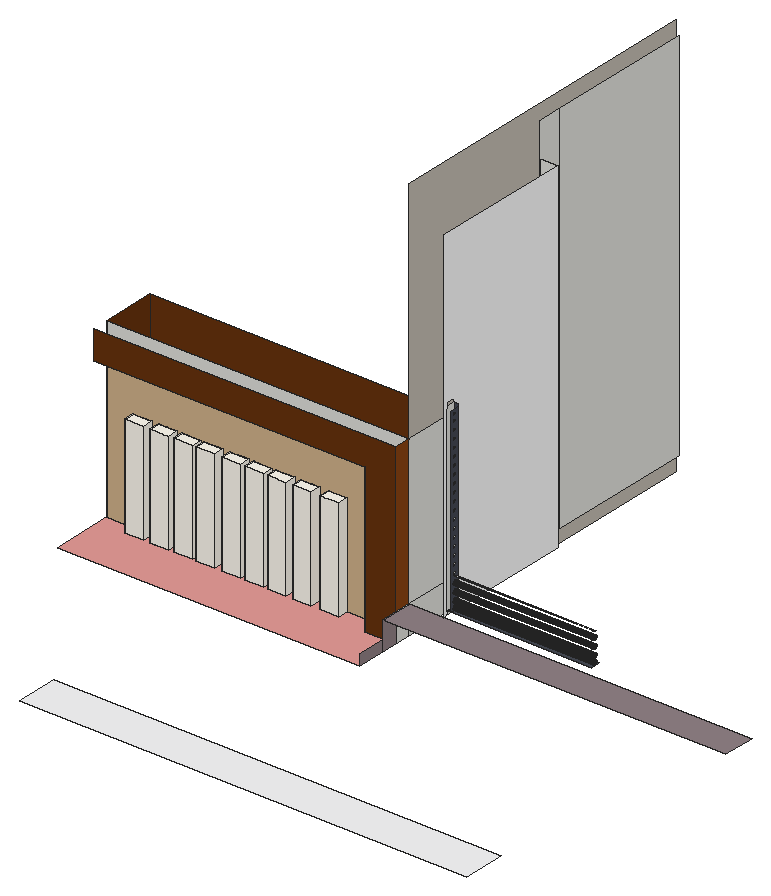
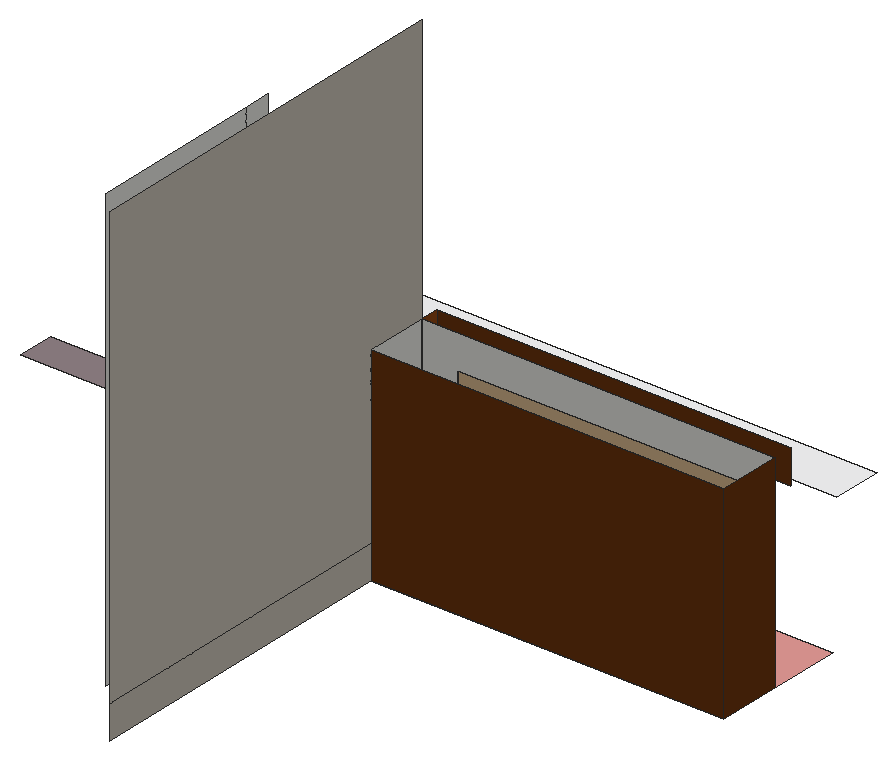
# SketchUp Ruby script. Lengths in inches.
U = 1.inch
M = Sketchup.active_model
def pt(a) = Geom::Point3d.new(a.map { |v| v * U })
def face(e, loops, mat)
  f = e.add_face(loops[0].map { |a| pt(a) })
  loops[1..].each { |l| e.add_face(l.map { |a| pt(a) }).erase! }
  f.material = f.back_material = mat if mat
  f
end
# faces: each face lists its corners as indices into pts; further lists are holes
def faces(e, pts, list, mat = nil) = list.each { |f| face(e, (f[0].is_a?(Array) ? f : [f]).map { |l| l.map { |i| pts[i] } }, mat) }
# xy, xz, yz: faces in a plane at the given z, y or x. An outline is a flat list of corners, or four numbers for a rectangle; further outlines are holes
def ring(l) = l.size == 4 ? [[l[0], l[1]], [l[2], l[1]], [l[2], l[3]], [l[0], l[3]]] : l.each_slice(2).to_a
def flat(e, list, mat, &to3) = list.each { |f| face(e, (f[0].is_a?(Array) ? f : [f]).map { |l| ring(l).map { |u, v| to3.(u, v) } }, mat) }
def xy(e, z, list, mat = nil) = flat(e, list, mat) { |x, y| [x, y, z] }
def xz(e, y, list, mat = nil) = flat(e, list, mat) { |x, z| [x, y, z] }
def yz(e, x, list, mat = nil) = flat(e, list, mat) { |y, z| [x, y, z] }
def lines(e, pts, list) = list.each { |a, b| e.add_line(pt(pts[a]), pt(pts[b])) }
# prism: a flat outline (further loops are holes) pulled along v
def prism(e, loops, v, mat = nil)
  f = face(e, loops, mat); d = Geom::Vector3d.new(v.map { |x| x * U })
  f.pushpull(f.normal.samedirection?(d) ? d.length : -d.length)
end
def box(e, o, s, mat = nil) = prism(e, [[o, [o[0] + s[0], o[1], o[2]], [o[0] + s[0], o[1] + s[1], o[2]], [o[0], o[1] + s[1], o[2]]]], [0, 0, s[2]], mat)
def at(x, y, z, deg = 0) = Geom::Transformation.translation(pt([x, y, z])) * Geom::Transformation.rotation(ORIGIN, Z_AXIS, deg.degrees)
def axes(o, x, y, z) = Geom::Transformation.new([*x, 0, *y, 0, *z, 0, *pt(o).to_a, 1])
def part(name) = M.definitions.add(name)
# library, detail: a bought-in or finely detailed component or shape, given as its bounding box
def library(name, o, s) = part(name).tap { |d| box(d.entities, o, s) }
def detail(e, o, s) = box(e.add_group.entities, o, s)
def put(e, d, t, mat = nil) = e.add_instance(d, t).tap { |i| i.material = mat if mat }
def group(e, t, mat = nil) = e.add_group.tap { |g| g.transformation = t; g.material = mat if mat }.entities
root = M.entities
M.materials.add("[0027_PeachPuff]").color = [255, 218, 185]
M.materials.add("[0035_Tan]").color = [210, 180, 140]
M.materials.add("[0043_SaddleBrown]").color = [104, 51, 14]
M.materials.add("[0043_SaddleBrown]1").color = [139, 69, 19]
M.materials.add("[0052_FloralWhite]").color = [255, 250, 240]
M.materials.add("[Asphalt New]").color = [145, 130, 134]
M.materials.add("[Brick Basket]").color = [230, 156, 152]
M.materials.add("[Field Rectangle Tile]").color = [196, 189, 179]
M.materials.add("[Formica Laminate Dark]").color = [70, 74, 84]
M.materials.add("[Polished Concrete New]").color = [200, 200, 203]
M.materials.add("[Quartz Light Grey]").color = [251, 251, 252]
xy(root,0,[[86.375,112.04,96.16,117.35],[8.39,113.98,14.33,117.35],[16.46,113.98,22.4,117.35],[23.96,113.98,29.9,117.35],[30.96,113.98,36.9,117.35],
  [39.27,113.98,45.21,117.35],[46.71,113.98,52.65,117.35],[53.83,113.98,59.77,117.35],[61.83,113.98,67.77,117.35],[70.58,113.98,76.52,117.35],
  [0,117.35,96.16,134.6]])
xy(root,0,[[0,97.66,0,117.35,8.39,117.35,8.39,113.98,14.33,113.98,14.33,117.35,16.46,117.35,16.46,113.98,22.4,113.98,22.4,117.35,23.96,117.35,23.96,113.98,29.9,113.98,29.9,117.35,30.96,117.35,30.96,113.98,36.9,113.98,36.9,117.35,39.27,117.35,39.27,113.98,45.21,113.98,45.21,117.35,46.71,117.35,46.71,113.98,52.65,113.98,52.65,117.35,53.83,117.35,53.83,113.98,59.77,113.98,59.77,117.35,61.83,117.35,61.83,113.98,67.77,113.98,67.77,117.35,70.58,117.35,70.58,113.98,76.52,113.98,76.52,117.35,86.375,117.35,86.375,112.04,96.16,112.04,96.16,97.66]],"[Brick Basket]")
xy(root,0,[[41.43,31,183.87,44.5]],"[Quartz Light Grey]")
xy(root,9,[[96.16,107.04,205.34,117.35]],"[Asphalt New]")
xy(root,10.25,[[107.21,118.87,108.27,121.64]])
xy(root,10.25,[[108.27,118.87,153.22,121.64]],"[Formica Laminate Dark]")
xy(root,32.4375,[[8.39,113.98,14.33,117.35],[16.46,113.98,22.4,117.35],[23.96,113.98,29.9,117.35],[30.96,113.98,36.9,117.35],[39.27,113.98,45.21,117.35],
  [46.71,113.98,52.65,117.35],[53.83,113.98,59.77,117.35],[61.83,113.98,67.77,117.35],[70.58,113.98,76.52,117.35]],"[0052_FloralWhite]")
xz(root,112.04,[[86.375,0,96.16,0,96.16,56.125,0,56.125,0,47.01,86.375,47.01]],"[0043_SaddleBrown]")
xz(root,113.98,[[8.39,0,14.33,32.4375],[16.46,0,22.4,32.4375],[23.96,0,29.9,32.4375],[30.96,0,36.9,32.4375],[39.27,0,45.21,32.4375],
  [46.71,0,52.65,32.4375],[53.83,0,59.77,32.4375],[61.83,0,67.77,32.4375],[70.58,0,76.52,32.4375]],"[0052_FloralWhite]")
xz(root,117.35,[[86.375,0,86.375,47.01,0,47.01,0,56.125,96.16,56.125,96.16,0],[8.39,0,14.33,32.4375],[16.46,0,22.4,32.4375],[23.96,0,29.9,32.4375],[30.96,0,36.9,32.4375],
  [39.27,0,45.21,32.4375],[46.71,0,52.65,32.4375],[53.83,0,59.77,32.4375],[61.83,0,67.77,32.4375],[70.58,0,76.52,32.4375]])
xz(root,117.35,[[0,0,8.39,0,8.39,32.4375,14.33,32.4375,14.33,0,16.46,0,16.46,32.4375,22.4,32.4375,22.4,0,23.96,0,23.96,32.4375,29.9,32.4375,29.9,0,30.96,0,30.96,32.4375,36.9,32.4375,36.9,0,39.27,0,39.27,32.4375,45.21,32.4375,45.21,0,46.71,0,46.71,32.4375,52.65,32.4375,52.65,0,53.83,0,53.83,32.4375,59.77,32.4375,59.77,0,61.83,0,61.83,32.4375,67.77,32.4375,67.77,0,70.58,0,70.58,32.4375,76.52,32.4375,76.52,0,86.375,0,86.375,47.01,0,47.01]],"[0035_Tan]")
xz(root,121.64,[[107.21,10.25,108.27,68.58]],"[Formica Laminate Dark]")
xz(root,134.6,[[0,0,96.16,56.125]],"[0043_SaddleBrown]")
xz(root,162.72,[[101.58,9,107.21,118.16]])
yz(root,0,[[117.35,0,134.6,56.125]],"[0043_SaddleBrown]")
yz(root,8.39,[[113.98,0,117.35,32.4375]],"[0052_FloralWhite]")
yz(root,14.33,[[113.98,0,117.35,32.4375]],"[0052_FloralWhite]")
yz(root,16.46,[[113.98,0,117.35,32.4375]],"[0052_FloralWhite]")
yz(root,22.4,[[113.98,0,117.35,32.4375]],"[0052_FloralWhite]")
yz(root,23.96,[[113.98,0,117.35,32.4375]],"[0052_FloralWhite]")
yz(root,29.9,[[113.98,0,117.35,32.4375]],"[0052_FloralWhite]")
yz(root,30.96,[[113.98,0,117.35,32.4375]],"[0052_FloralWhite]")
yz(root,36.9,[[113.98,0,117.35,32.4375]],"[0052_FloralWhite]")
yz(root,39.27,[[113.98,0,117.35,32.4375]],"[0052_FloralWhite]")
yz(root,45.21,[[113.98,0,117.35,32.4375]],"[0052_FloralWhite]")
yz(root,46.71,[[113.98,0,117.35,32.4375]],"[0052_FloralWhite]")
yz(root,52.65,[[113.98,0,117.35,32.4375]],"[0052_FloralWhite]")
yz(root,53.83,[[113.98,0,117.35,32.4375]],"[0052_FloralWhite]")
yz(root,59.77,[[113.98,0,117.35,32.4375]],"[0052_FloralWhite]")
yz(root,61.83,[[113.98,0,117.35,32.4375]],"[0052_FloralWhite]")
yz(root,67.77,[[113.98,0,117.35,32.4375]],"[0052_FloralWhite]")
yz(root,70.58,[[113.98,0,117.35,32.4375]],"[0052_FloralWhite]")
yz(root,76.52,[[113.98,0,117.35,32.4375]],"[0052_FloralWhite]")
yz(root,86.375,[[112.04,0,117.35,47.01]],"[0027_PeachPuff]")
yz(root,96.16,[[112.04,0,117.35,9],[117.35,0,134.6,9],[117.35,9,134.6,56.125]])
yz(root,96.16,[[112.04,9,117.35,56.125]],"[0043_SaddleBrown]1")
yz(root,96.16,[[97.66,0,107.04,3.4375],[107.04,0,112.04,9]],"[Asphalt New]")
yz(root,96.16,[[134.6,0,223.51,9],[134.6,9,134.6,56.125,117.35,56.125,117.35,129,223.51,129,223.51,9]],"[Field Rectangle Tile]")
yz(root,101.58,[[162.72,9,170.43,129],[170.43,9,218.08,129]])
yz(root,107.21,[[118.87,9,121.64,10.25],[118.87,10.25,121.64,68.58]])
yz(root,107.21,[[117.35,9,118.87,9,118.87,69.75,121.64,69.75,121.64,9,162.72,9,162.72,118.16,117.35,118.16]],"[Quartz Light Grey]")
yz(root,108.27,[[120.22,9.91,120.38,9.93,120.53,9.99,120.66,10.09,120.76,10.22,120.77,10.25,119.67,10.25,119.68,10.22,119.78,10.09,119.91,9.99,120.06,9.93],[120.22,10.47,120.06,10.49,119.91,10.56,119.78,10.66,119.68,10.79,119.61,10.9375,119.59,11.1,119.61,11.26,119.68,11.41,119.78,11.54,119.91,11.64,120.06,11.7,120.22,11.72,120.38,11.7,120.53,11.64,120.66,11.54,120.76,11.41,120.82,11.26,120.84,11.1,120.82,10.9375,120.76,10.79,120.66,10.66,120.53,10.56,120.38,10.49],[120.22,12.47,120.06,12.49,119.91,12.56,119.78,12.66,119.68,12.79,119.61,12.9375,119.59,13.1,119.61,13.26,119.68,13.41,119.78,13.54,119.91,13.64,120.06,13.7,120.22,13.72,120.38,13.7,120.53,13.64,120.66,13.54,120.76,13.41,120.82,13.26,120.84,13.1,120.82,12.9375,120.76,12.79,120.66,12.66,120.53,12.56,120.38,12.49],[120.22,15.04,120.06,15.06,119.91,15.12,119.78,15.22,119.68,15.35,119.61,15.5,119.59,15.66,119.61,15.82,119.68,15.97,119.78,16.1,119.91,16.2,120.06,16.26,120.22,16.29,120.38,16.26,120.53,16.2,120.66,16.1,120.76,15.97,120.82,15.82,120.84,15.66,120.82,15.5,120.76,15.35,120.66,15.22,120.53,15.12,120.38,15.06],[120.22,17.6,120.06,17.62,119.91,17.68,119.78,17.78,119.68,17.91,119.61,18.0625,119.59,18.22,119.61,18.38,119.68,18.54,119.78,18.66,119.91,18.76,120.06,18.83,120.22,18.85,120.38,18.83,120.53,18.76,120.66,18.66,120.76,18.54,120.82,18.38,120.84,18.22,120.82,18.0625,120.76,17.91,120.66,17.78,120.53,17.68,120.38,17.62],
  [120.22,20.16,120.06,20.18,119.91,20.24,119.78,20.34,119.68,20.47,119.61,20.625,119.59,20.79,119.61,20.95,119.68,21.1,119.78,21.23,119.91,21.33,120.06,21.39,120.22,21.41,120.38,21.39,120.53,21.33,120.66,21.23,120.76,21.1,120.82,20.95,120.84,20.79,120.82,20.625,120.76,20.47,120.66,20.34,120.53,20.24,120.38,20.18],[120.22,22.72,120.06,22.74,119.91,22.81,119.78,22.91,119.68,23.04,119.61,23.1875,119.59,23.35,119.61,23.51,119.68,23.66,119.78,23.79,119.91,23.89,120.06,23.95,120.22,23.97,120.38,23.95,120.53,23.89,120.66,23.79,120.76,23.66,120.82,23.51,120.84,23.35,120.82,23.1875,120.76,23.04,120.66,22.91,120.53,22.81,120.38,22.74],[120.22,25.29,120.06,25.31,119.91,25.37,119.78,25.47,119.68,25.6,119.61,25.75,119.59,25.91,119.61,26.07,119.68,26.22,119.78,26.35,119.91,26.45,120.06,26.51,120.22,26.54,120.38,26.51,120.53,26.45,120.66,26.35,120.76,26.22,120.82,26.07,120.84,25.91,120.82,25.75,120.76,25.6,120.66,25.47,120.53,25.37,120.38,25.31],[120.22,27.85,120.06,27.87,119.91,27.93,119.78,28.03,119.68,28.16,119.61,28.3125,119.59,28.47,119.61,28.63,119.68,28.79,119.78,28.91,119.91,29.01,120.06,29.08,120.22,29.1,120.38,29.08,120.53,29.01,120.66,28.91,120.76,28.79,120.82,28.63,120.84,28.47,120.82,28.3125,120.76,28.16,120.66,28.03,120.53,27.93,120.38,27.87],[120.22,30.41,120.06,30.43,119.91,30.49,119.78,30.59,119.68,30.72,119.61,30.875,119.59,31.04,119.61,31.2,119.68,31.35,119.78,31.48,119.91,31.58,120.06,31.64,120.22,31.66,120.38,31.64,120.53,31.58,120.66,31.48,120.76,31.35,120.82,31.2,120.84,31.04,120.82,30.875,120.76,30.72,120.66,30.59,120.53,30.49,120.38,30.43],
  [120.22,32.97,120.06,32.99,119.91,33.06,119.78,33.16,119.68,33.29,119.61,33.4375,119.59,33.6,119.61,33.76,119.68,33.91,119.78,34.04,119.91,34.14,120.06,34.2,120.22,34.22,120.38,34.2,120.53,34.14,120.66,34.04,120.76,33.91,120.82,33.76,120.84,33.6,120.82,33.4375,120.76,33.29,120.66,33.16,120.53,33.06,120.38,32.99],[120.22,35.54,120.06,35.56,119.91,35.62,119.78,35.72,119.68,35.85,119.61,36,119.59,36.16,119.61,36.32,119.68,36.47,119.78,36.6,119.91,36.7,120.06,36.76,120.22,36.79,120.38,36.76,120.53,36.7,120.66,36.6,120.76,36.47,120.82,36.32,120.84,36.16,120.82,36,120.76,35.85,120.66,35.72,120.53,35.62,120.38,35.56]])
yz(root,108.27,[[[118.87,10.25,121.64,67.58],[120.22,15.04,120.06,15.06,119.91,15.12,119.78,15.22,119.68,15.35,119.61,15.5,119.59,15.66,119.61,15.82,119.68,15.97,119.78,16.1,119.91,16.2,120.06,16.26,120.22,16.29,120.38,16.26,120.53,16.2,120.66,16.1,120.76,15.97,120.82,15.82,120.84,15.66,120.82,15.5,120.76,15.35,120.66,15.22,120.53,15.12,120.38,15.06],[120.22,63.72,120.06,63.74,119.91,63.81,119.78,63.91,119.68,64.04,119.61,64.1875,119.59,64.35,119.61,64.51,119.68,64.66,119.78,64.79,119.91,64.89,120.06,64.95,120.22,64.97,120.38,64.95,120.53,64.89,120.66,64.79,120.76,64.66,120.82,64.51,120.84,64.35,120.82,64.1875,120.76,64.04,120.66,63.91,120.53,63.81,120.38,63.74],[120.22,65.6,120.06,65.62,119.91,65.68,119.78,65.78,119.68,65.91,119.61,66.0625,119.59,66.22,119.61,66.38,119.68,66.54,119.78,66.66,119.91,66.76,120.06,66.83,120.22,66.85,120.38,66.83,120.53,66.76,120.66,66.66,120.76,66.54,120.82,66.38,120.84,66.22,120.82,66.0625,120.76,65.91,120.66,65.78,120.53,65.68,120.38,65.62],[120.22,61.16,120.06,61.18,119.91,61.24,119.78,61.34,119.68,61.47,119.61,61.625,119.59,61.79,119.61,61.95,119.68,62.1,119.78,62.23,119.91,62.33,120.06,62.39,120.22,62.41,120.38,62.39,120.53,62.33,120.66,62.23,120.76,62.1,120.82,61.95,120.84,61.79,120.82,61.625,120.76,61.47,120.66,61.34,120.53,61.24,120.38,61.18],[120.22,58.6,120.06,58.62,119.91,58.68,119.78,58.78,119.68,58.91,119.61,59.0625,119.59,59.22,119.61,59.38,119.68,59.54,119.78,59.66,119.91,59.76,120.06,59.83,120.22,59.85,120.38,59.83,120.53,59.76,120.66,59.66,120.76,59.54,120.82,59.38,120.84,59.22,120.82,59.0625,120.76,58.91,120.66,58.78,120.53,58.68,120.38,58.62],[120.22,56.04,120.06,56.06,119.91,56.12,119.78,56.22,119.68,56.35,119.61,56.5,119.59,56.66,119.61,56.82,119.68,56.97,119.78,57.1,119.91,57.2,120.06,57.26,120.22,57.29,120.38,57.26,120.53,57.2,120.66,57.1,120.76,56.97,120.82,56.82,120.84,56.66,120.82,56.5,120.76,56.35,120.66,56.22,120.53,56.12,120.38,56.06],[120.22,53.47,120.06,53.49,119.91,53.56,119.78,53.66,119.68,53.79,119.61,53.9375,119.59,54.1,119.61,54.26,119.68,54.41,119.78,54.54,119.91,54.64,120.06,54.7,120.22,54.72,120.38,54.7,120.53,54.64,120.66,54.54,120.76,54.41,120.82,54.26,120.84,54.1,120.82,53.9375,120.76,53.79,120.66,53.66,120.53,53.56,120.38,53.49],[120.22,50.91,120.06,50.93,119.91,50.99,119.78,51.09,119.68,51.22,119.61,51.375,119.59,51.54,119.61,51.7,119.68,51.85,119.78,51.98,119.91,52.08,120.06,52.14,120.22,52.16,120.38,52.14,120.53,52.08,120.66,51.98,120.76,51.85,120.82,51.7,120.84,51.54,120.82,51.375,120.76,51.22,120.66,51.09,120.53,50.99,120.38,50.93],[120.22,48.35,120.06,48.37,119.91,48.43,119.78,48.53,119.68,48.66,119.61,48.8125,119.59,48.97,119.61,49.13,119.68,49.29,119.78,49.41,119.91,49.51,120.06,49.58,120.22,49.6,120.38,49.58,120.53,49.51,120.66,49.41,120.76,49.29,120.82,49.13,120.84,48.97,120.82,48.8125,120.76,48.66,120.66,48.53,120.53,48.43,120.38,48.37],[120.22,45.79,120.06,45.81,119.91,45.87,119.78,45.97,119.68,46.1,119.61,46.25,119.59,46.41,119.61,46.57,119.68,46.72,119.78,46.85,119.91,46.95,120.06,47.01,120.22,47.04,120.38,47.01,120.53,46.95,120.66,46.85,120.76,46.72,120.82,46.57,120.84,46.41,120.82,46.25,120.76,46.1,120.66,45.97,120.53,45.87,120.38,45.81],[120.22,43.22,120.06,43.24,119.91,43.31,119.78,43.41,119.68,43.54,119.61,43.6875,119.59,43.85,119.61,44.01,119.68,44.16,119.78,44.29,119.91,44.39,120.06,44.45,120.22,44.47,120.38,44.45,120.53,44.39,120.66,44.29,120.76,44.16,120.82,44.01,120.84,43.85,120.82,43.6875,120.76,43.54,120.66,43.41,120.53,43.31,120.38,43.24],[120.22,40.66,120.06,40.68,119.91,40.74,119.78,40.84,119.68,40.97,119.61,41.125,119.59,41.29,119.61,41.45,119.68,41.6,119.78,41.73,119.91,41.83,120.06,41.89,120.22,41.91,120.38,41.89,120.53,41.83,120.66,41.73,120.76,41.6,120.82,41.45,120.84,41.29,120.82,41.125,120.76,40.97,120.66,40.84,120.53,40.74,120.38,40.68],[120.22,38.1,120.06,38.12,119.91,38.18,119.78,38.28,119.68,38.41,119.61,38.5625,119.59,38.72,119.61,38.88,119.68,39.04,119.78,39.16,119.91,39.26,120.06,39.33,120.22,39.35,120.38,39.33,120.53,39.26,120.66,39.16,120.76,39.04,120.82,38.88,120.84,38.72,120.82,38.5625,120.76,38.41,120.66,38.28,120.53,38.18,120.38,38.12],[120.22,35.54,120.06,35.56,119.91,35.62,119.78,35.72,119.68,35.85,119.61,36,119.59,36.16,119.61,36.32,119.68,36.47,119.78,36.6,119.91,36.7,120.06,36.76,120.22,36.79,120.38,36.76,120.53,36.7,120.66,36.6,120.76,36.47,120.82,36.32,120.84,36.16,120.82,36,120.76,35.85,120.66,35.72,120.53,35.62,120.38,35.56],[120.22,32.97,120.06,32.99,119.91,33.06,119.78,33.16,119.68,33.29,119.61,33.4375,119.59,33.6,119.61,33.76,119.68,33.91,119.78,34.04,119.91,34.14,120.06,34.2,120.22,34.22,120.38,34.2,120.53,34.14,120.66,34.04,120.76,33.91,120.82,33.76,120.84,33.6,120.82,33.4375,120.76,33.29,120.66,33.16,120.53,33.06,120.38,32.99],[120.22,30.41,120.06,30.43,119.91,30.49,119.78,30.59,119.68,30.72,119.61,30.875,119.59,31.04,119.61,31.2,119.68,31.35,119.78,31.48,119.91,31.58,120.06,31.64,120.22,31.66,120.38,31.64,120.53,31.58,120.66,31.48,120.76,31.35,120.82,31.2,120.84,31.04,120.82,30.875,120.76,30.72,120.66,30.59,120.53,30.49,120.38,30.43],[120.22,27.85,120.06,27.87,119.91,27.93,119.78,28.03,119.68,28.16,119.61,28.3125,119.59,28.47,119.61,28.63,119.68,28.79,119.78,28.91,119.91,29.01,120.06,29.08,120.22,29.1,120.38,29.08,120.53,29.01,120.66,28.91,120.76,28.79,120.82,28.63,120.84,28.47,120.82,28.3125,120.76,28.16,120.66,28.03,120.53,27.93,120.38,27.87],[120.22,25.29,120.06,25.31,119.91,25.37,119.78,25.47,119.68,25.6,119.61,25.75,119.59,25.91,119.61,26.07,119.68,26.22,119.78,26.35,119.91,26.45,120.06,26.51,120.22,26.54,120.38,26.51,120.53,26.45,120.66,26.35,120.76,26.22,120.82,26.07,120.84,25.91,120.82,25.75,120.76,25.6,120.66,25.47,120.53,25.37,120.38,25.31],[120.22,22.72,120.06,22.74,119.91,22.81,119.78,22.91,119.68,23.04,119.61,23.1875,119.59,23.35,119.61,23.51,119.68,23.66,119.78,23.79,119.91,23.89,120.06,23.95,120.22,23.97,120.38,23.95,120.53,23.89,120.66,23.79,120.76,23.66,120.82,23.51,120.84,23.35,120.82,23.1875,120.76,23.04,120.66,22.91,120.53,22.81,120.38,22.74],[120.22,20.16,120.06,20.18,119.91,20.24,119.78,20.34,119.68,20.47,119.61,20.625,119.59,20.79,119.61,20.95,119.68,21.1,119.78,21.23,119.91,21.33,120.06,21.39,120.22,21.41,120.38,21.39,120.53,21.33,120.66,21.23,120.76,21.1,120.82,20.95,120.84,20.79,120.82,20.625,120.76,20.47,120.66,20.34,120.53,20.24,120.38,20.18],[120.22,17.6,120.06,17.62,119.91,17.68,119.78,17.78,119.68,17.91,119.61,18.0625,119.59,18.22,119.61,18.38,119.68,18.54,119.78,18.66,119.91,18.76,120.06,18.83,120.22,18.85,120.38,18.83,120.53,18.76,120.66,18.66,120.76,18.54,120.82,18.38,120.84,18.22,120.82,18.0625,120.76,17.91,120.66,17.78,120.53,17.68,120.38,17.62],[120.22,12.47,120.06,12.49,119.91,12.56,119.78,12.66,119.68,12.79,119.61,12.9375,119.59,13.1,119.61,13.26,119.68,13.41,119.78,13.54,119.91,13.64,120.06,13.7,120.22,13.72,120.38,13.7,120.53,13.64,120.66,13.54,120.76,13.41,120.82,13.26,120.84,13.1,120.82,12.9375,120.76,12.79,120.66,12.66,120.53,12.56,120.38,12.49],[120.22,10.47,120.06,10.49,119.91,10.56,119.78,10.66,119.68,10.79,119.61,10.9375,119.59,11.1,119.61,11.26,119.68,11.41,119.78,11.54,119.91,11.64,120.06,11.7,120.22,11.72,120.38,11.7,120.53,11.64,120.66,11.54,120.76,11.41,120.82,11.26,120.84,11.1,120.82,10.9375,120.76,10.79,120.66,10.66,120.53,10.56,120.38,10.49]]],"[Formica Laminate Dark]")
p = [[108.27,119.91,10.56],[108.27,120.06,10.49],[153.22,120.06,10.49],[153.22,119.91,10.56],[108.27,120.22,10.47],[153.22,120.22,10.47],
  [108.27,120.38,10.49],[153.22,120.38,10.49],[108.27,120.53,10.56],[153.22,120.53,10.56],[108.27,119.78,10.66],[153.22,119.78,10.66],
  [108.27,120.66,10.66],[153.22,120.66,10.66],[108.27,119.68,10.79],[153.22,119.68,10.79],[108.27,120.76,10.79],[153.22,120.76,10.79],
  [108.27,119.61,10.9375],[153.22,119.61,10.9375],[108.27,120.82,10.9375],[153.22,120.82,10.9375],[108.27,119.59,11.1],[153.22,119.59,11.1],
  [108.27,120.84,11.1],[153.22,120.84,11.1],[108.27,119.61,11.26],[153.22,119.61,11.26],[108.27,120.82,11.26],[153.22,120.82,11.26],
  [108.27,119.68,11.41],[153.22,119.68,11.41],[108.27,120.76,11.41],[153.22,120.76,11.41],[108.27,119.78,11.54],[153.22,119.78,11.54],
  [108.27,120.66,11.54],[153.22,120.66,11.54],[108.27,119.91,11.64],[153.22,119.91,11.64],[108.27,120.53,11.64],[153.22,120.53,11.64],
  [108.27,120.06,11.7],[153.22,120.06,11.7],[108.27,120.38,11.7],[153.22,120.38,11.7],[108.27,120.22,11.72],[153.22,120.22,11.72],
  [108.27,119.91,12.56],[108.27,120.06,12.49],[153.22,120.06,12.49],[153.22,119.91,12.56],[108.27,120.22,12.47],[153.22,120.22,12.47],
  [108.27,120.38,12.49],[153.22,120.38,12.49],[108.27,120.53,12.56],[153.22,120.53,12.56],[108.27,119.78,12.66],[153.22,119.78,12.66],
  [108.27,120.66,12.66],[153.22,120.66,12.66],[108.27,119.68,12.79],[153.22,119.68,12.79],[108.27,120.76,12.79],[153.22,120.76,12.79],
  [108.27,119.61,12.9375],[153.22,119.61,12.9375],[108.27,120.82,12.9375],[153.22,120.82,12.9375],[108.27,119.59,13.1],[153.22,119.59,13.1],
  [108.27,120.84,13.1],[153.22,120.84,13.1],[108.27,119.61,13.26],[153.22,119.61,13.26],[108.27,120.82,13.26],[153.22,120.82,13.26],
  [108.27,119.68,13.41],[153.22,119.68,13.41],[108.27,120.76,13.41],[153.22,120.76,13.41],[108.27,119.78,13.54],[153.22,119.78,13.54],
  [108.27,120.66,13.54],[153.22,120.66,13.54],[108.27,119.91,13.64],[153.22,119.91,13.64],[108.27,120.53,13.64],[153.22,120.53,13.64],
  [108.27,120.06,13.7],[153.22,120.06,13.7],[108.27,120.38,13.7],[153.22,120.38,13.7],[108.27,120.22,13.72],[153.22,120.22,13.72],
  [108.27,120.06,15.06],[108.27,120.22,15.04],[153.22,120.22,15.04],[153.22,120.06,15.06],[108.27,120.38,15.06],[153.22,120.38,15.06],
  [108.27,119.78,15.22],[108.27,119.91,15.12],[153.22,119.91,15.12],[153.22,119.78,15.22],[108.27,120.53,15.12],[153.22,120.53,15.12],
  [108.27,120.66,15.22],[153.22,120.66,15.22],[108.27,119.68,15.35],[153.22,119.68,15.35],[108.27,120.76,15.35],[153.22,120.76,15.35],
  [108.27,119.61,15.5],[153.22,119.61,15.5],[108.27,120.82,15.5],[153.22,120.82,15.5],[108.27,119.59,15.66],[153.22,119.59,15.66],
  [108.27,120.84,15.66],[153.22,120.84,15.66],[108.27,119.61,15.82],[153.22,119.61,15.82],[108.27,120.82,15.82],[153.22,120.82,15.82],
  [108.27,119.68,15.97],[153.22,119.68,15.97],[108.27,120.76,15.97],[153.22,120.76,15.97],[108.27,119.78,16.1],[153.22,119.78,16.1],
  [108.27,120.66,16.1],[153.22,120.66,16.1],[108.27,119.91,16.2],[153.22,119.91,16.2],[108.27,120.53,16.2],[153.22,120.53,16.2],
  [108.27,120.06,16.26],[153.22,120.06,16.26],[108.27,120.38,16.26],[153.22,120.38,16.26],[108.27,120.22,16.29],[153.22,120.22,16.29],
  [108.27,119.91,17.68],[108.27,120.06,17.62],[153.22,120.06,17.62],[153.22,119.91,17.68],[108.27,120.22,17.6],[153.22,120.22,17.6],
  [108.27,120.38,17.62],[153.22,120.38,17.62],[108.27,120.53,17.68],[153.22,120.53,17.68],[108.27,119.78,17.78],[153.22,119.78,17.78],
  [108.27,120.66,17.78],[153.22,120.66,17.78],[108.27,119.68,17.91],[153.22,119.68,17.91],[108.27,120.76,17.91],[153.22,120.76,17.91],
  [108.27,119.61,18.0625],[153.22,119.61,18.0625],[108.27,120.82,18.0625],[153.22,120.82,18.0625],[108.27,119.59,18.22],[153.22,119.59,18.22],
  [108.27,120.84,18.22],[153.22,120.84,18.22],[108.27,119.61,18.38],[153.22,119.61,18.38],[108.27,120.82,18.38],[153.22,120.82,18.38],
  [108.27,119.68,18.54],[153.22,119.68,18.54],[108.27,120.76,18.54],[153.22,120.76,18.54],[108.27,119.78,18.66],[153.22,119.78,18.66],
  [108.27,120.66,18.66],[153.22,120.66,18.66],[108.27,119.91,18.76],[153.22,119.91,18.76],[108.27,120.53,18.76],[153.22,120.53,18.76],
  [108.27,120.06,18.83],[153.22,120.06,18.83],[108.27,120.22,18.85],[153.22,120.22,18.85],[108.27,120.38,18.83],[153.22,120.38,18.83],
  [108.27,120.06,20.18],[108.27,120.22,20.16],[153.22,120.22,20.16],[153.22,120.06,20.18],[108.27,120.38,20.18],[153.22,120.38,20.18]]
faces(root,p,[[0,1,2,3],[1,4,5,2],[4,6,7,5],[6,8,9,7],[10,0,3,11],[8,12,13,9],[14,10,11,15],[12,16,17,13],
  [18,14,15,19],[16,20,21,17],[22,18,19,23],[20,24,25,21],[26,22,23,27],[24,28,29,25],[30,26,27,31],[28,32,33,29],
  [34,30,31,35],[32,36,37,33],[38,34,35,39],[36,40,41,37],[42,38,39,43],[40,44,45,41],[46,42,43,47],[44,46,47,45],
  [48,49,50,51],[49,52,53,50],[52,54,55,53],[54,56,57,55],[58,48,51,59],[56,60,61,57],[62,58,59,63],[60,64,65,61],
  [66,62,63,67],[64,68,69,65],[70,66,67,71],[68,72,73,69],[74,70,71,75],[72,76,77,73],[78,74,75,79],[76,80,81,77],
  [82,78,79,83],[80,84,85,81],[86,82,83,87],[84,88,89,85],[90,86,87,91],[88,92,93,89],[94,90,91,95],[92,94,95,93],
  [96,97,98,99],[97,100,101,98],[102,103,104,105],[103,96,99,104],[100,106,107,101],[106,108,109,107],[110,102,105,111],[108,112,113,109],
  [114,110,111,115],[112,116,117,113],[118,114,115,119],[116,120,121,117],[122,118,119,123],[120,124,125,121],[126,122,123,127],[124,128,129,125],
  [130,126,127,131],[128,132,133,129],[134,130,131,135],[132,136,137,133],[138,134,135,139],[136,140,141,137],[142,138,139,143],[140,142,143,141],
  [144,145,146,147],[145,148,149,146],[148,150,151,149],[150,152,153,151],[154,144,147,155],[152,156,157,153],[158,154,155,159],[156,160,161,157],
  [162,158,159,163],[160,164,165,161],[166,162,163,167],[164,168,169,165],[170,166,167,171],[168,172,173,169],[174,170,171,175],[172,176,177,173],
  [178,174,175,179],[176,180,181,177],[182,178,179,183],[180,184,185,181],[186,182,183,187],[188,186,187,189],[190,188,189,191],[184,190,191,185],
  [192,193,194,195],[193,196,197,194]],"[Polished Concrete New]")
